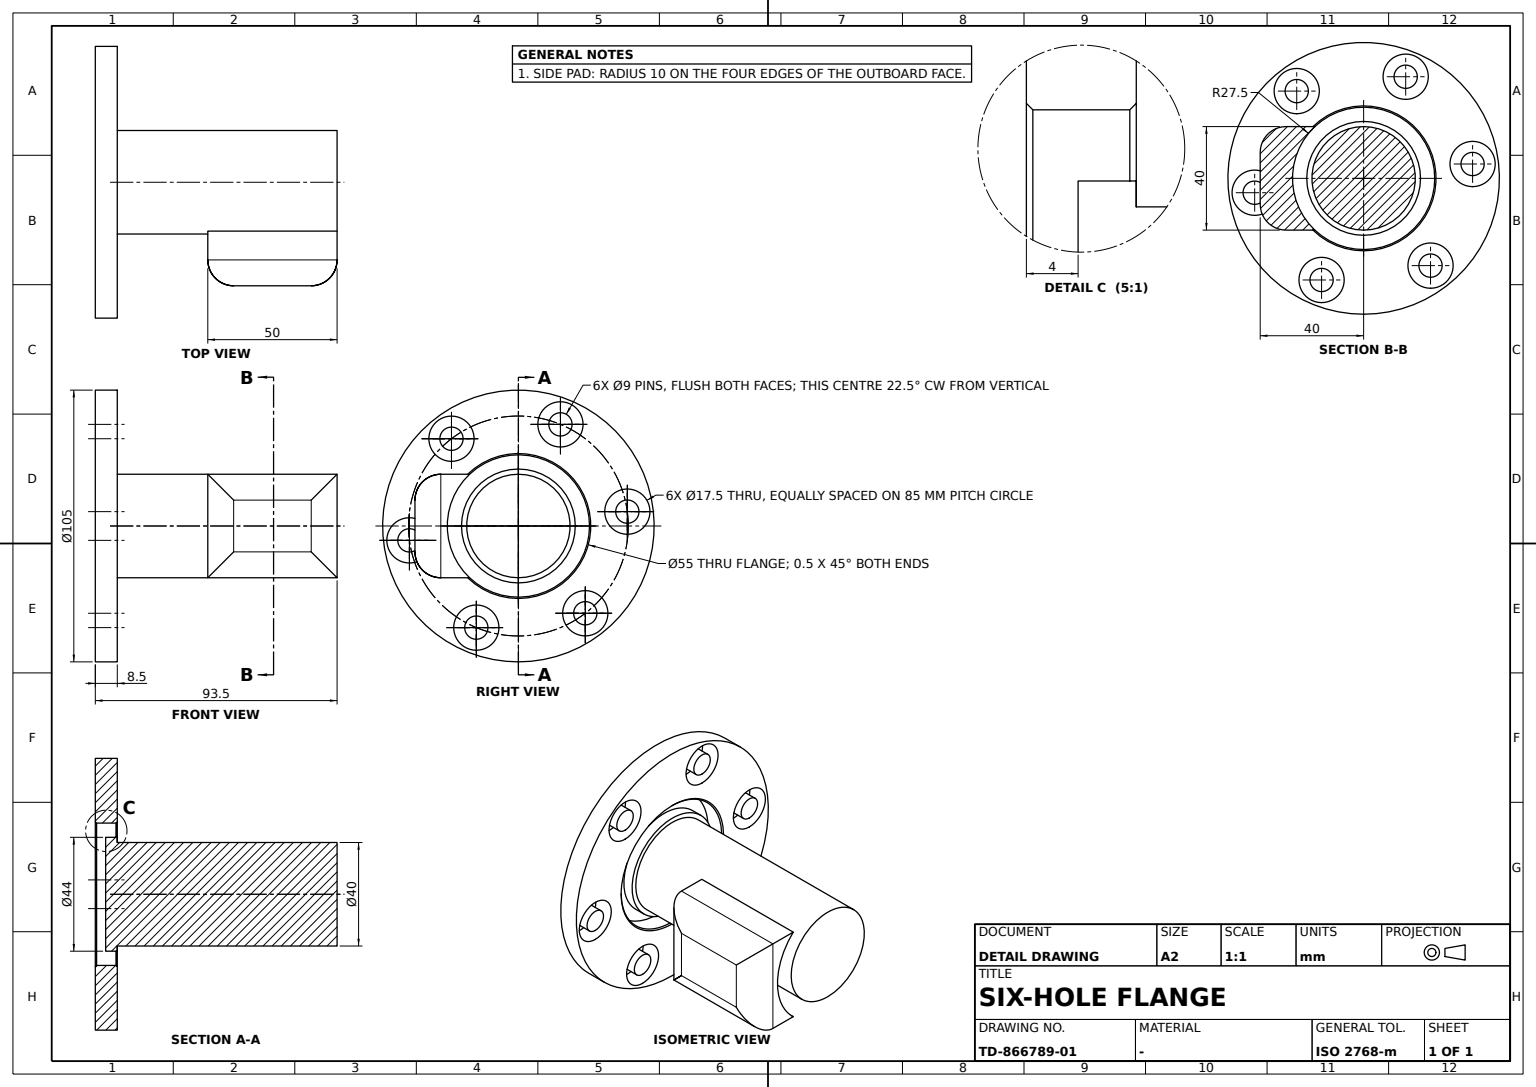
ISO-10303-21;
HEADER;
FILE_DESCRIPTION((''),'2;1');
FILE_NAME('','',(''),(''),'','','');
FILE_SCHEMA(('AUTOMOTIVE_DESIGN'));
ENDSEC;
DATA;
#1=APPLICATION_CONTEXT('');
#2=PRODUCT_CONTEXT('',#1,'mechanical');
#3=PRODUCT('','','',(#2));
#4=PRODUCT_DEFINITION_FORMATION('','',#3);
#5=PRODUCT_DEFINITION_CONTEXT('',#1,'design');
#6=PRODUCT_DEFINITION('','',#4,#5);
#7=PRODUCT_DEFINITION_SHAPE('','',#6);
#8=(LENGTH_UNIT()NAMED_UNIT(*)SI_UNIT(.MILLI.,.METRE.));
#9=(NAMED_UNIT(*)PLANE_ANGLE_UNIT()SI_UNIT($,.RADIAN.));
#10=(NAMED_UNIT(*)SI_UNIT($,.STERADIAN.)SOLID_ANGLE_UNIT());
#11=UNCERTAINTY_MEASURE_WITH_UNIT(LENGTH_MEASURE(0.005),#8,'distance_accuracy_value','');
#12=(GEOMETRIC_REPRESENTATION_CONTEXT(3)GLOBAL_UNCERTAINTY_ASSIGNED_CONTEXT((#11))GLOBAL_UNIT_ASSIGNED_CONTEXT((#8,#9,#10))REPRESENTATION_CONTEXT('',''));
#13=CARTESIAN_POINT('',(-1.047363,42.136407,0.));
#14=VERTEX_POINT('',#13);
#15=CARTESIAN_POINT('',(-5.547363,42.136407,0.));
#16=DIRECTION('',(0.,0.,1.));
#17=DIRECTION('',(1.,0.,0.));
#18=AXIS2_PLACEMENT_3D('',#15,#16,#17);
#19=CIRCLE('',#18,4.5);
#20=EDGE_CURVE('',#14,#14,#19,.T.);
#21=ORIENTED_EDGE('',*,*,#20,.T.);
#22=EDGE_LOOP('',(#21));
#23=FACE_BOUND('',#22,.T.);
#24=CARTESIAN_POINT('',(-1.047363,42.136407,8.5));
#25=VERTEX_POINT('',#24);
#26=CARTESIAN_POINT('',(-5.547363,42.136407,8.5));
#27=AXIS2_PLACEMENT_3D('',#26,#16,#17);
#28=CIRCLE('',#27,4.5);
#29=EDGE_CURVE('',#25,#25,#28,.T.);
#30=ORIENTED_EDGE('',*,*,#29,.F.);
#31=EDGE_LOOP('',(#30));
#32=FACE_BOUND('',#31,.T.);
#33=CARTESIAN_POINT('',(-5.547363,42.136407,4.25));
#34=AXIS2_PLACEMENT_3D('',#33,#16,#17);
#35=CYLINDRICAL_SURFACE('',#34,4.5);
#36=ADVANCED_FACE('',(#23,#32),#35,.T.);
#37=ORIENTED_EDGE('',*,*,#20,.F.);
#38=EDGE_LOOP('',(#37));
#39=FACE_BOUND('',#38,.T.);
#40=CARTESIAN_POINT('',(0.,0.,0.));
#41=AXIS2_PLACEMENT_3D('',#40,#16,#17);
#42=PLANE('',#41);
#43=ADVANCED_FACE('',(#39),#42,.F.);
#44=ORIENTED_EDGE('',*,*,#29,.T.);
#45=EDGE_LOOP('',(#44));
#46=FACE_BOUND('',#45,.T.);
#47=CARTESIAN_POINT('',(0.,0.,8.5));
#48=AXIS2_PLACEMENT_3D('',#47,#16,#17);
#49=PLANE('',#48);
#50=ADVANCED_FACE('',(#46),#49,.T.);
#51=CLOSED_SHELL('',(#36,#43,#50));
#52=MANIFOLD_SOLID_BREP('',#51);
#53=CARTESIAN_POINT('',(52.5,0.,8.5));
#54=VERTEX_POINT('',#53);
#55=CIRCLE('',#48,52.5);
#56=EDGE_CURVE('',#54,#54,#55,.T.);
#57=ORIENTED_EDGE('',*,*,#56,.F.);
#58=EDGE_LOOP('',(#57));
#59=FACE_BOUND('',#58,.T.);
#60=CARTESIAN_POINT('',(52.5,0.,0.));
#61=VERTEX_POINT('',#60);
#62=CIRCLE('',#41,52.5);
#63=EDGE_CURVE('',#61,#61,#62,.T.);
#64=ORIENTED_EDGE('',*,*,#63,.T.);
#65=EDGE_LOOP('',(#64));
#66=FACE_BOUND('',#65,.T.);
#67=CARTESIAN_POINT('',(0.,0.,4.25));
#68=AXIS2_PLACEMENT_3D('',#67,#16,#17);
#69=CYLINDRICAL_SURFACE('',#68,52.5);
#70=ADVANCED_FACE('',(#59,#66),#69,.T.);
#71=CARTESIAN_POINT('',(-30.51488,16.264046,8.5));
#72=VERTEX_POINT('',#71);
#73=CARTESIAN_POINT('',(-39.26488,16.264046,8.5));
#74=AXIS2_PLACEMENT_3D('',#73,#16,#17);
#75=CIRCLE('',#74,8.75);
#76=EDGE_CURVE('',#72,#72,#75,.T.);
#77=ORIENTED_EDGE('',*,*,#76,.T.);
#78=EDGE_LOOP('',(#77));
#79=FACE_BOUND('',#78,.T.);
#80=CARTESIAN_POINT('',(-30.51488,16.264046,0.));
#81=VERTEX_POINT('',#80);
#82=CARTESIAN_POINT('',(-39.26488,16.264046,0.));
#83=AXIS2_PLACEMENT_3D('',#82,#16,#17);
#84=CIRCLE('',#83,8.75);
#85=EDGE_CURVE('',#81,#81,#84,.T.);
#86=ORIENTED_EDGE('',*,*,#85,.F.);
#87=EDGE_LOOP('',(#86));
#88=FACE_BOUND('',#87,.T.);
#89=CARTESIAN_POINT('',(-39.26488,16.264046,4.25));
#90=AXIS2_PLACEMENT_3D('',#89,#16,#17);
#91=CYLINDRICAL_SURFACE('',#90,8.75);
#92=ADVANCED_FACE('',(#79,#88),#91,.F.);
#93=CARTESIAN_POINT('',(0.,-27.5,8.));
#94=VERTEX_POINT('',#93);
#95=CARTESIAN_POINT('',(0.,0.,8.));
#96=DIRECTION('',(0.,-1.,0.));
#97=AXIS2_PLACEMENT_3D('',#95,#16,#96);
#98=CIRCLE('',#97,27.5);
#99=EDGE_CURVE('',#94,#94,#98,.T.);
#100=ORIENTED_EDGE('',*,*,#99,.F.);
#101=EDGE_LOOP('',(#100));
#102=FACE_BOUND('',#101,.T.);
#103=CARTESIAN_POINT('',(28.,0.,8.5));
#104=VERTEX_POINT('',#103);
#105=CIRCLE('',#48,28.);
#106=EDGE_CURVE('',#104,#104,#105,.T.);
#107=ORIENTED_EDGE('',*,*,#106,.T.);
#108=EDGE_LOOP('',(#107));
#109=FACE_BOUND('',#108,.T.);
#110=CARTESIAN_POINT('',(0.,0.,-19.5));
#111=DIRECTION('',(-0.904494219,0.426485883,0.));
#112=AXIS2_PLACEMENT_3D('',#110,#16,#111);
#113=CONICAL_SURFACE('',#112,0.,0.785398163);
#114=ADVANCED_FACE('',(#102,#109),#113,.F.);
#115=ORIENTED_EDGE('',*,*,#56,.T.);
#116=EDGE_LOOP('',(#115));
#117=FACE_BOUND('',#116,.T.);
#118=CARTESIAN_POINT('',(48.01488,-16.264046,8.5));
#119=VERTEX_POINT('',#118);
#120=CARTESIAN_POINT('',(39.26488,-16.264046,8.5));
#121=AXIS2_PLACEMENT_3D('',#120,#16,#17);
#122=CIRCLE('',#121,8.75);
#123=EDGE_CURVE('',#119,#119,#122,.T.);
#124=ORIENTED_EDGE('',*,*,#123,.F.);
#125=EDGE_LOOP('',(#124));
#126=FACE_BOUND('',#125,.T.);
#127=CARTESIAN_POINT('',(3.202637,42.136407,8.5));
#128=VERTEX_POINT('',#127);
#129=CIRCLE('',#27,8.75);
#130=EDGE_CURVE('',#128,#128,#129,.T.);
#131=ORIENTED_EDGE('',*,*,#130,.F.);
#132=EDGE_LOOP('',(#131));
#133=FACE_BOUND('',#132,.T.);
#134=CARTESIAN_POINT('',(14.297363,-42.136407,8.5));
#135=VERTEX_POINT('',#134);
#136=CARTESIAN_POINT('',(5.547363,-42.136407,8.5));
#137=AXIS2_PLACEMENT_3D('',#136,#16,#17);
#138=CIRCLE('',#137,8.75);
#139=EDGE_CURVE('',#135,#135,#138,.T.);
#140=ORIENTED_EDGE('',*,*,#139,.F.);
#141=EDGE_LOOP('',(#140));
#142=FACE_BOUND('',#141,.T.);
#143=ORIENTED_EDGE('',*,*,#76,.F.);
#144=EDGE_LOOP('',(#143));
#145=FACE_BOUND('',#144,.T.);
#146=ORIENTED_EDGE('',*,*,#106,.F.);
#147=EDGE_LOOP('',(#146));
#148=FACE_BOUND('',#147,.T.);
#149=CARTESIAN_POINT('',(42.467517,25.872361,8.5));
#150=VERTEX_POINT('',#149);
#151=CARTESIAN_POINT('',(33.717517,25.872361,8.5));
#152=AXIS2_PLACEMENT_3D('',#151,#16,#17);
#153=CIRCLE('',#152,8.75);
#154=EDGE_CURVE('',#150,#150,#153,.T.);
#155=ORIENTED_EDGE('',*,*,#154,.F.);
#156=EDGE_LOOP('',(#155));
#157=FACE_BOUND('',#156,.T.);
#158=CARTESIAN_POINT('',(-24.967517,-25.872361,8.5));
#159=VERTEX_POINT('',#158);
#160=CARTESIAN_POINT('',(-33.717517,-25.872361,8.5));
#161=AXIS2_PLACEMENT_3D('',#160,#16,#17);
#162=CIRCLE('',#161,8.75);
#163=EDGE_CURVE('',#159,#159,#162,.T.);
#164=ORIENTED_EDGE('',*,*,#163,.F.);
#165=EDGE_LOOP('',(#164));
#166=FACE_BOUND('',#165,.T.);
#167=ADVANCED_FACE('',(#117,#126,#133,#142,#145,#148,#157,#166),#49,.T.);
#168=ORIENTED_EDGE('',*,*,#163,.T.);
#169=EDGE_LOOP('',(#168));
#170=FACE_BOUND('',#169,.T.);
#171=CARTESIAN_POINT('',(-24.967517,-25.872361,0.));
#172=VERTEX_POINT('',#171);
#173=CARTESIAN_POINT('',(-33.717517,-25.872361,0.));
#174=AXIS2_PLACEMENT_3D('',#173,#16,#17);
#175=CIRCLE('',#174,8.75);
#176=EDGE_CURVE('',#172,#172,#175,.T.);
#177=ORIENTED_EDGE('',*,*,#176,.F.);
#178=EDGE_LOOP('',(#177));
#179=FACE_BOUND('',#178,.T.);
#180=CARTESIAN_POINT('',(-33.717517,-25.872361,4.25));
#181=AXIS2_PLACEMENT_3D('',#180,#16,#17);
#182=CYLINDRICAL_SURFACE('',#181,8.75);
#183=ADVANCED_FACE('',(#170,#179),#182,.F.);
#184=ORIENTED_EDGE('',*,*,#130,.T.);
#185=EDGE_LOOP('',(#184));
#186=FACE_BOUND('',#185,.T.);
#187=CARTESIAN_POINT('',(3.202637,42.136407,0.));
#188=VERTEX_POINT('',#187);
#189=CIRCLE('',#18,8.75);
#190=EDGE_CURVE('',#188,#188,#189,.T.);
#191=ORIENTED_EDGE('',*,*,#190,.F.);
#192=EDGE_LOOP('',(#191));
#193=FACE_BOUND('',#192,.T.);
#194=CYLINDRICAL_SURFACE('',#34,8.75);
#195=ADVANCED_FACE('',(#186,#193),#194,.F.);
#196=CARTESIAN_POINT('',(48.01488,-16.264046,0.));
#197=VERTEX_POINT('',#196);
#198=CARTESIAN_POINT('',(39.26488,-16.264046,0.));
#199=AXIS2_PLACEMENT_3D('',#198,#16,#17);
#200=CIRCLE('',#199,8.75);
#201=EDGE_CURVE('',#197,#197,#200,.T.);
#202=ORIENTED_EDGE('',*,*,#201,.F.);
#203=EDGE_LOOP('',(#202));
#204=FACE_BOUND('',#203,.T.);
#205=ORIENTED_EDGE('',*,*,#123,.T.);
#206=EDGE_LOOP('',(#205));
#207=FACE_BOUND('',#206,.T.);
#208=CARTESIAN_POINT('',(39.26488,-16.264046,4.25));
#209=AXIS2_PLACEMENT_3D('',#208,#16,#17);
#210=CYLINDRICAL_SURFACE('',#209,8.75);
#211=ADVANCED_FACE('',(#204,#207),#210,.F.);
#212=ORIENTED_EDGE('',*,*,#190,.T.);
#213=EDGE_LOOP('',(#212));
#214=FACE_BOUND('',#213,.T.);
#215=ORIENTED_EDGE('',*,*,#85,.T.);
#216=EDGE_LOOP('',(#215));
#217=FACE_BOUND('',#216,.T.);
#218=ORIENTED_EDGE('',*,*,#63,.F.);
#219=EDGE_LOOP('',(#218));
#220=FACE_BOUND('',#219,.T.);
#221=ORIENTED_EDGE('',*,*,#201,.T.);
#222=EDGE_LOOP('',(#221));
#223=FACE_BOUND('',#222,.T.);
#224=CARTESIAN_POINT('',(42.467517,25.872361,0.));
#225=VERTEX_POINT('',#224);
#226=CARTESIAN_POINT('',(33.717517,25.872361,0.));
#227=AXIS2_PLACEMENT_3D('',#226,#16,#17);
#228=CIRCLE('',#227,8.75);
#229=EDGE_CURVE('',#225,#225,#228,.T.);
#230=ORIENTED_EDGE('',*,*,#229,.T.);
#231=EDGE_LOOP('',(#230));
#232=FACE_BOUND('',#231,.T.);
#233=CARTESIAN_POINT('',(28.,0.,0.));
#234=VERTEX_POINT('',#233);
#235=CIRCLE('',#41,28.);
#236=EDGE_CURVE('',#234,#234,#235,.T.);
#237=ORIENTED_EDGE('',*,*,#236,.T.);
#238=EDGE_LOOP('',(#237));
#239=FACE_BOUND('',#238,.T.);
#240=CARTESIAN_POINT('',(14.297363,-42.136407,0.));
#241=VERTEX_POINT('',#240);
#242=CARTESIAN_POINT('',(5.547363,-42.136407,0.));
#243=AXIS2_PLACEMENT_3D('',#242,#16,#17);
#244=CIRCLE('',#243,8.75);
#245=EDGE_CURVE('',#241,#241,#244,.T.);
#246=ORIENTED_EDGE('',*,*,#245,.T.);
#247=EDGE_LOOP('',(#246));
#248=FACE_BOUND('',#247,.T.);
#249=ORIENTED_EDGE('',*,*,#176,.T.);
#250=EDGE_LOOP('',(#249));
#251=FACE_BOUND('',#250,.T.);
#252=ADVANCED_FACE('',(#214,#217,#220,#223,#232,#239,#248,#251),#42,.F.);
#253=ORIENTED_EDGE('',*,*,#236,.F.);
#254=EDGE_LOOP('',(#253));
#255=FACE_BOUND('',#254,.T.);
#256=CARTESIAN_POINT('',(0.,27.5,0.5));
#257=VERTEX_POINT('',#256);
#258=CARTESIAN_POINT('',(0.,0.,0.5));
#259=DIRECTION('',(0.,0.,-1.));
#260=DIRECTION('',(0.,1.,0.));
#261=AXIS2_PLACEMENT_3D('',#258,#259,#260);
#262=CIRCLE('',#261,27.5);
#263=EDGE_CURVE('',#257,#257,#262,.F.);
#264=ORIENTED_EDGE('',*,*,#263,.T.);
#265=EDGE_LOOP('',(#264));
#266=FACE_BOUND('',#265,.T.);
#267=CARTESIAN_POINT('',(0.,0.,28.));
#268=DIRECTION('',(0.904494219,-0.426485883,0.));
#269=AXIS2_PLACEMENT_3D('',#267,#259,#268);
#270=CONICAL_SURFACE('',#269,0.,0.785398163);
#271=ADVANCED_FACE('',(#255,#266),#270,.F.);
#272=ORIENTED_EDGE('',*,*,#229,.F.);
#273=EDGE_LOOP('',(#272));
#274=FACE_BOUND('',#273,.T.);
#275=ORIENTED_EDGE('',*,*,#154,.T.);
#276=EDGE_LOOP('',(#275));
#277=FACE_BOUND('',#276,.T.);
#278=CARTESIAN_POINT('',(33.717517,25.872361,4.25));
#279=AXIS2_PLACEMENT_3D('',#278,#16,#17);
#280=CYLINDRICAL_SURFACE('',#279,8.75);
#281=ADVANCED_FACE('',(#274,#277),#280,.F.);
#282=ORIENTED_EDGE('',*,*,#263,.F.);
#283=EDGE_LOOP('',(#282));
#284=FACE_BOUND('',#283,.T.);
#285=ORIENTED_EDGE('',*,*,#99,.T.);
#286=EDGE_LOOP('',(#285));
#287=FACE_BOUND('',#286,.T.);
#288=CYLINDRICAL_SURFACE('',#68,27.5);
#289=ADVANCED_FACE('',(#284,#287),#288,.F.);
#290=ORIENTED_EDGE('',*,*,#139,.T.);
#291=EDGE_LOOP('',(#290));
#292=FACE_BOUND('',#291,.T.);
#293=ORIENTED_EDGE('',*,*,#245,.F.);
#294=EDGE_LOOP('',(#293));
#295=FACE_BOUND('',#294,.T.);
#296=CARTESIAN_POINT('',(5.547363,-42.136407,4.25));
#297=AXIS2_PLACEMENT_3D('',#296,#16,#17);
#298=CYLINDRICAL_SURFACE('',#297,8.75);
#299=ADVANCED_FACE('',(#292,#295),#298,.F.);
#300=CLOSED_SHELL('',(#70,#92,#114,#167,#183,#195,#211,#252,#271,#281,#289,#299));
#301=MANIFOLD_SOLID_BREP('',#300);
#302=CARTESIAN_POINT('',(22.,0.,4.));
#303=VERTEX_POINT('',#302);
#304=CARTESIAN_POINT('',(0.,0.,4.));
#305=AXIS2_PLACEMENT_3D('',#304,#16,#17);
#306=CIRCLE('',#305,22.);
#307=EDGE_CURVE('',#303,#303,#306,.T.);
#308=ORIENTED_EDGE('',*,*,#307,.T.);
#309=EDGE_LOOP('',(#308));
#310=FACE_BOUND('',#309,.T.);
#311=CARTESIAN_POINT('',(22.,0.,8.5));
#312=VERTEX_POINT('',#311);
#313=CIRCLE('',#48,22.);
#314=EDGE_CURVE('',#312,#312,#313,.T.);
#315=ORIENTED_EDGE('',*,*,#314,.F.);
#316=EDGE_LOOP('',(#315));
#317=FACE_BOUND('',#316,.T.);
#318=CYLINDRICAL_SURFACE('',#68,22.);
#319=ADVANCED_FACE('',(#310,#317),#318,.T.);
#320=CARTESIAN_POINT('',(20.,0.,93.5));
#321=VERTEX_POINT('',#320);
#322=CARTESIAN_POINT('',(0.,0.,93.5));
#323=AXIS2_PLACEMENT_3D('',#322,#16,#17);
#324=CIRCLE('',#323,20.);
#325=EDGE_CURVE('',#321,#321,#324,.T.);
#326=ORIENTED_EDGE('',*,*,#325,.T.);
#327=EDGE_LOOP('',(#326));
#328=FACE_BOUND('',#327,.T.);
#329=PLANE('',#323);
#330=ADVANCED_FACE('',(#328),#329,.T.);
#331=ORIENTED_EDGE('',*,*,#314,.T.);
#332=EDGE_LOOP('',(#331));
#333=FACE_BOUND('',#332,.T.);
#334=CARTESIAN_POINT('',(20.,0.,8.5));
#335=VERTEX_POINT('',#334);
#336=CIRCLE('',#48,20.);
#337=EDGE_CURVE('',#335,#335,#336,.T.);
#338=ORIENTED_EDGE('',*,*,#337,.F.);
#339=EDGE_LOOP('',(#338));
#340=FACE_BOUND('',#339,.T.);
#341=ADVANCED_FACE('',(#333,#340),#49,.T.);
#342=ORIENTED_EDGE('',*,*,#337,.T.);
#343=EDGE_LOOP('',(#342));
#344=FACE_BOUND('',#343,.T.);
#345=ORIENTED_EDGE('',*,*,#325,.F.);
#346=EDGE_LOOP('',(#345));
#347=FACE_BOUND('',#346,.T.);
#348=CARTESIAN_POINT('',(0.,0.,51.));
#349=AXIS2_PLACEMENT_3D('',#348,#16,#17);
#350=CYLINDRICAL_SURFACE('',#349,20.);
#351=ADVANCED_FACE('',(#344,#347),#350,.T.);
#352=ORIENTED_EDGE('',*,*,#307,.F.);
#353=EDGE_LOOP('',(#352));
#354=FACE_BOUND('',#353,.T.);
#355=CARTESIAN_POINT('',(-1.616457,0.,4.));
#356=AXIS2_PLACEMENT_3D('',#355,#16,#17);
#357=PLANE('',#356);
#358=ADVANCED_FACE('',(#354),#357,.F.);
#359=CLOSED_SHELL('',(#319,#330,#341,#351,#358));
#360=MANIFOLD_SOLID_BREP('',#359);
#361=CARTESIAN_POINT('',(38.217517,25.872361,0.));
#362=VERTEX_POINT('',#361);
#363=CIRCLE('',#227,4.5);
#364=EDGE_CURVE('',#362,#362,#363,.T.);
#365=ORIENTED_EDGE('',*,*,#364,.F.);
#366=EDGE_LOOP('',(#365));
#367=FACE_BOUND('',#366,.T.);
#368=ADVANCED_FACE('',(#367),#42,.F.);
#369=CARTESIAN_POINT('',(38.217517,25.872361,8.5));
#370=VERTEX_POINT('',#369);
#371=CIRCLE('',#152,4.5);
#372=EDGE_CURVE('',#370,#370,#371,.T.);
#373=ORIENTED_EDGE('',*,*,#372,.T.);
#374=EDGE_LOOP('',(#373));
#375=FACE_BOUND('',#374,.T.);
#376=ADVANCED_FACE('',(#375),#49,.T.);
#377=ORIENTED_EDGE('',*,*,#364,.T.);
#378=EDGE_LOOP('',(#377));
#379=FACE_BOUND('',#378,.T.);
#380=ORIENTED_EDGE('',*,*,#372,.F.);
#381=EDGE_LOOP('',(#380));
#382=FACE_BOUND('',#381,.T.);
#383=CYLINDRICAL_SURFACE('',#279,4.5);
#384=ADVANCED_FACE('',(#379,#382),#383,.T.);
#385=CLOSED_SHELL('',(#368,#376,#384));
#386=MANIFOLD_SOLID_BREP('',#385);
#387=CARTESIAN_POINT('',(43.76488,-16.264046,8.5));
#388=VERTEX_POINT('',#387);
#389=CIRCLE('',#121,4.5);
#390=EDGE_CURVE('',#388,#388,#389,.T.);
#391=ORIENTED_EDGE('',*,*,#390,.F.);
#392=EDGE_LOOP('',(#391));
#393=FACE_BOUND('',#392,.T.);
#394=CARTESIAN_POINT('',(43.76488,-16.264046,0.));
#395=VERTEX_POINT('',#394);
#396=CIRCLE('',#199,4.5);
#397=EDGE_CURVE('',#395,#395,#396,.T.);
#398=ORIENTED_EDGE('',*,*,#397,.T.);
#399=EDGE_LOOP('',(#398));
#400=FACE_BOUND('',#399,.T.);
#401=CYLINDRICAL_SURFACE('',#209,4.5);
#402=ADVANCED_FACE('',(#393,#400),#401,.T.);
#403=ORIENTED_EDGE('',*,*,#390,.T.);
#404=EDGE_LOOP('',(#403));
#405=FACE_BOUND('',#404,.T.);
#406=ADVANCED_FACE('',(#405),#49,.T.);
#407=ORIENTED_EDGE('',*,*,#397,.F.);
#408=EDGE_LOOP('',(#407));
#409=FACE_BOUND('',#408,.T.);
#410=ADVANCED_FACE('',(#409),#42,.F.);
#411=CLOSED_SHELL('',(#402,#406,#410));
#412=MANIFOLD_SOLID_BREP('',#411);
#413=CARTESIAN_POINT('',(10.047363,-42.136407,8.5));
#414=VERTEX_POINT('',#413);
#415=CIRCLE('',#137,4.5);
#416=EDGE_CURVE('',#414,#414,#415,.T.);
#417=ORIENTED_EDGE('',*,*,#416,.T.);
#418=EDGE_LOOP('',(#417));
#419=FACE_BOUND('',#418,.T.);
#420=ADVANCED_FACE('',(#419),#49,.T.);
#421=ORIENTED_EDGE('',*,*,#416,.F.);
#422=EDGE_LOOP('',(#421));
#423=FACE_BOUND('',#422,.T.);
#424=CARTESIAN_POINT('',(10.047363,-42.136407,0.));
#425=VERTEX_POINT('',#424);
#426=CIRCLE('',#243,4.5);
#427=EDGE_CURVE('',#425,#425,#426,.T.);
#428=ORIENTED_EDGE('',*,*,#427,.T.);
#429=EDGE_LOOP('',(#428));
#430=FACE_BOUND('',#429,.T.);
#431=CYLINDRICAL_SURFACE('',#297,4.5);
#432=ADVANCED_FACE('',(#423,#430),#431,.T.);
#433=ORIENTED_EDGE('',*,*,#427,.F.);
#434=EDGE_LOOP('',(#433));
#435=FACE_BOUND('',#434,.T.);
#436=ADVANCED_FACE('',(#435),#42,.F.);
#437=CLOSED_SHELL('',(#420,#432,#436));
#438=MANIFOLD_SOLID_BREP('',#437);
#439=CARTESIAN_POINT('',(-29.217517,-25.872361,0.));
#440=VERTEX_POINT('',#439);
#441=CIRCLE('',#174,4.5);
#442=EDGE_CURVE('',#440,#440,#441,.T.);
#443=ORIENTED_EDGE('',*,*,#442,.T.);
#444=EDGE_LOOP('',(#443));
#445=FACE_BOUND('',#444,.T.);
#446=CARTESIAN_POINT('',(-29.217517,-25.872361,8.5));
#447=VERTEX_POINT('',#446);
#448=CIRCLE('',#161,4.5);
#449=EDGE_CURVE('',#447,#447,#448,.T.);
#450=ORIENTED_EDGE('',*,*,#449,.F.);
#451=EDGE_LOOP('',(#450));
#452=FACE_BOUND('',#451,.T.);
#453=CYLINDRICAL_SURFACE('',#181,4.5);
#454=ADVANCED_FACE('',(#445,#452),#453,.T.);
#455=ORIENTED_EDGE('',*,*,#449,.T.);
#456=EDGE_LOOP('',(#455));
#457=FACE_BOUND('',#456,.T.);
#458=ADVANCED_FACE('',(#457),#49,.T.);
#459=ORIENTED_EDGE('',*,*,#442,.F.);
#460=EDGE_LOOP('',(#459));
#461=FACE_BOUND('',#460,.T.);
#462=ADVANCED_FACE('',(#461),#42,.F.);
#463=CLOSED_SHELL('',(#454,#458,#462));
#464=MANIFOLD_SOLID_BREP('',#463);
#465=CARTESIAN_POINT('',(-34.76488,16.264046,8.5));
#466=VERTEX_POINT('',#465);
#467=CIRCLE('',#74,4.5);
#468=EDGE_CURVE('',#466,#466,#467,.T.);
#469=ORIENTED_EDGE('',*,*,#468,.T.);
#470=EDGE_LOOP('',(#469));
#471=FACE_BOUND('',#470,.T.);
#472=ADVANCED_FACE('',(#471),#49,.T.);
#473=CARTESIAN_POINT('',(-34.76488,16.264046,0.));
#474=VERTEX_POINT('',#473);
#475=CIRCLE('',#83,4.5);
#476=EDGE_CURVE('',#474,#474,#475,.T.);
#477=ORIENTED_EDGE('',*,*,#476,.T.);
#478=EDGE_LOOP('',(#477));
#479=FACE_BOUND('',#478,.T.);
#480=ORIENTED_EDGE('',*,*,#468,.F.);
#481=EDGE_LOOP('',(#480));
#482=FACE_BOUND('',#481,.T.);
#483=CYLINDRICAL_SURFACE('',#90,4.5);
#484=ADVANCED_FACE('',(#479,#482),#483,.T.);
#485=ORIENTED_EDGE('',*,*,#476,.F.);
#486=EDGE_LOOP('',(#485));
#487=FACE_BOUND('',#486,.T.);
#488=ADVANCED_FACE('',(#487),#42,.F.);
#489=CLOSED_SHELL('',(#472,#484,#488));
#490=MANIFOLD_SOLID_BREP('',#489);
#491=CARTESIAN_POINT('',(-10.,-40.,53.5));
#492=VERTEX_POINT('',#491);
#493=CARTESIAN_POINT('',(-20.,-30.,43.5));
#494=VERTEX_POINT('',#493);
#495=CARTESIAN_POINT('',(-10.,-30.,53.5));
#496=DIRECTION('',(0.707106781,0.,-0.707106781));
#497=DIRECTION('',(0.707106781,0.,0.707106781));
#498=AXIS2_PLACEMENT_3D('',#495,#496,#497);
#499=ELLIPSE('',#498,14.142136,10.);
#500=EDGE_CURVE('',#492,#494,#499,.T.);
#501=ORIENTED_EDGE('',*,*,#500,.T.);
#502=CARTESIAN_POINT('',(20.,-30.,43.5));
#503=VERTEX_POINT('',#502);
#504=CARTESIAN_POINT('',(0.,-30.,43.5));
#505=VECTOR('',#17,1000.);
#506=LINE('',#504,#505);
#507=EDGE_CURVE('',#494,#503,#506,.T.);
#508=ORIENTED_EDGE('',*,*,#507,.T.);
#509=CARTESIAN_POINT('',(10.,-40.,53.5));
#510=VERTEX_POINT('',#509);
#511=CARTESIAN_POINT('',(10.,-30.,53.5));
#512=DIRECTION('',(-0.707106781,0.,-0.707106781));
#513=AXIS2_PLACEMENT_3D('',#511,#512,#496);
#514=ELLIPSE('',#513,14.142136,10.);
#515=EDGE_CURVE('',#510,#503,#514,.F.);
#516=ORIENTED_EDGE('',*,*,#515,.F.);
#517=CARTESIAN_POINT('',(0.,-40.,53.5));
#518=LINE('',#517,#505);
#519=EDGE_CURVE('',#492,#510,#518,.T.);
#520=ORIENTED_EDGE('',*,*,#519,.F.);
#521=EDGE_LOOP('',(#501,#508,#516,#520));
#522=FACE_BOUND('',#521,.T.);
#523=CARTESIAN_POINT('',(0.,-30.,53.5));
#524=AXIS2_PLACEMENT_3D('',#523,#17,#96);
#525=CYLINDRICAL_SURFACE('',#524,10.);
#526=ADVANCED_FACE('',(#522),#525,.T.);
#527=CARTESIAN_POINT('',(20.,-18.874586,43.5));
#528=VERTEX_POINT('',#527);
#529=VECTOR('',#96,1000.);
#530=LINE('',#527,#529);
#531=EDGE_CURVE('',#528,#503,#530,.T.);
#532=ORIENTED_EDGE('',*,*,#531,.T.);
#533=ORIENTED_EDGE('',*,*,#507,.F.);
#534=CARTESIAN_POINT('',(-20.,-18.874586,43.5));
#535=VERTEX_POINT('',#534);
#536=CARTESIAN_POINT('',(-20.,-40.,43.5));
#537=VECTOR('',#260,1000.);
#538=LINE('',#536,#537);
#539=EDGE_CURVE('',#494,#535,#538,.T.);
#540=ORIENTED_EDGE('',*,*,#539,.T.);
#541=CARTESIAN_POINT('',(0.,0.,43.5));
#542=AXIS2_PLACEMENT_3D('',#541,#16,#17);
#543=CIRCLE('',#542,27.5);
#544=EDGE_CURVE('',#535,#528,#543,.T.);
#545=ORIENTED_EDGE('',*,*,#544,.T.);
#546=EDGE_LOOP('',(#532,#533,#540,#545));
#547=FACE_BOUND('',#546,.T.);
#548=PLANE('',#542);
#549=ADVANCED_FACE('',(#547),#548,.F.);
#550=CARTESIAN_POINT('',(-20.,-30.,93.5));
#551=VERTEX_POINT('',#550);
#552=CARTESIAN_POINT('',(-20.,-18.874586,93.5));
#553=VERTEX_POINT('',#552);
#554=CARTESIAN_POINT('',(-20.,-40.,93.5));
#555=LINE('',#554,#537);
#556=EDGE_CURVE('',#551,#553,#555,.T.);
#557=ORIENTED_EDGE('',*,*,#556,.F.);
#558=CARTESIAN_POINT('',(20.,-30.,93.5));
#559=VERTEX_POINT('',#558);
#560=CARTESIAN_POINT('',(0.,-30.,93.5));
#561=LINE('',#560,#505);
#562=EDGE_CURVE('',#551,#559,#561,.T.);
#563=ORIENTED_EDGE('',*,*,#562,.T.);
#564=CARTESIAN_POINT('',(20.,-18.874586,93.5));
#565=VERTEX_POINT('',#564);
#566=LINE('',#564,#529);
#567=EDGE_CURVE('',#565,#559,#566,.T.);
#568=ORIENTED_EDGE('',*,*,#567,.F.);
#569=CIRCLE('',#323,27.5);
#570=EDGE_CURVE('',#553,#565,#569,.T.);
#571=ORIENTED_EDGE('',*,*,#570,.F.);
#572=EDGE_LOOP('',(#557,#563,#568,#571));
#573=FACE_BOUND('',#572,.T.);
#574=ADVANCED_FACE('',(#573),#329,.T.);
#575=ORIENTED_EDGE('',*,*,#500,.F.);
#576=CARTESIAN_POINT('',(-10.,-40.,83.5));
#577=VERTEX_POINT('',#576);
#578=CARTESIAN_POINT('',(-10.,-40.,68.5));
#579=VECTOR('',#259,1000.);
#580=LINE('',#578,#579);
#581=EDGE_CURVE('',#577,#492,#580,.T.);
#582=ORIENTED_EDGE('',*,*,#581,.F.);
#583=CARTESIAN_POINT('',(-10.,-30.,83.5));
#584=AXIS2_PLACEMENT_3D('',#583,#512,#496);
#585=ELLIPSE('',#584,14.142136,10.);
#586=EDGE_CURVE('',#577,#551,#585,.T.);
#587=ORIENTED_EDGE('',*,*,#586,.T.);
#588=CARTESIAN_POINT('',(-20.,-30.,68.5));
#589=LINE('',#588,#579);
#590=EDGE_CURVE('',#551,#494,#589,.T.);
#591=ORIENTED_EDGE('',*,*,#590,.T.);
#592=EDGE_LOOP('',(#575,#582,#587,#591));
#593=FACE_BOUND('',#592,.T.);
#594=CARTESIAN_POINT('',(-10.,-30.,68.5));
#595=AXIS2_PLACEMENT_3D('',#594,#259,#96);
#596=CYLINDRICAL_SURFACE('',#595,10.);
#597=ADVANCED_FACE('',(#593),#596,.T.);
#598=ORIENTED_EDGE('',*,*,#539,.F.);
#599=ORIENTED_EDGE('',*,*,#590,.F.);
#600=ORIENTED_EDGE('',*,*,#556,.T.);
#601=VECTOR('',#16,1000.);
#602=LINE('',#552,#601);
#603=EDGE_CURVE('',#553,#535,#602,.F.);
#604=ORIENTED_EDGE('',*,*,#603,.T.);
#605=EDGE_LOOP('',(#598,#599,#600,#604));
#606=FACE_BOUND('',#605,.T.);
#607=DIRECTION('',(-1.,0.,0.));
#608=AXIS2_PLACEMENT_3D('',#554,#607,#260);
#609=PLANE('',#608);
#610=ADVANCED_FACE('',(#606),#609,.T.);
#611=CARTESIAN_POINT('',(10.,-40.,83.5));
#612=VERTEX_POINT('',#611);
#613=CARTESIAN_POINT('',(10.,-30.,83.5));
#614=AXIS2_PLACEMENT_3D('',#613,#496,#497);
#615=ELLIPSE('',#614,14.142136,10.);
#616=EDGE_CURVE('',#612,#559,#615,.F.);
#617=ORIENTED_EDGE('',*,*,#616,.T.);
#618=ORIENTED_EDGE('',*,*,#562,.F.);
#619=ORIENTED_EDGE('',*,*,#586,.F.);
#620=CARTESIAN_POINT('',(0.,-40.,83.5));
#621=LINE('',#620,#505);
#622=EDGE_CURVE('',#577,#612,#621,.T.);
#623=ORIENTED_EDGE('',*,*,#622,.T.);
#624=EDGE_LOOP('',(#617,#618,#619,#623));
#625=FACE_BOUND('',#624,.T.);
#626=CARTESIAN_POINT('',(0.,-30.,83.5));
#627=AXIS2_PLACEMENT_3D('',#626,#17,#96);
#628=CYLINDRICAL_SURFACE('',#627,10.);
#629=ADVANCED_FACE('',(#625),#628,.T.);
#630=LINE('',#564,#601);
#631=EDGE_CURVE('',#565,#528,#630,.F.);
#632=ORIENTED_EDGE('',*,*,#631,.T.);
#633=ORIENTED_EDGE('',*,*,#544,.F.);
#634=ORIENTED_EDGE('',*,*,#603,.F.);
#635=ORIENTED_EDGE('',*,*,#570,.T.);
#636=EDGE_LOOP('',(#632,#633,#634,#635));
#637=FACE_BOUND('',#636,.T.);
#638=ADVANCED_FACE('',(#637),#288,.F.);
#639=ORIENTED_EDGE('',*,*,#616,.F.);
#640=CARTESIAN_POINT('',(10.,-40.,68.5));
#641=LINE('',#640,#579);
#642=EDGE_CURVE('',#612,#510,#641,.T.);
#643=ORIENTED_EDGE('',*,*,#642,.T.);
#644=ORIENTED_EDGE('',*,*,#515,.T.);
#645=CARTESIAN_POINT('',(20.,-30.,68.5));
#646=LINE('',#645,#579);
#647=EDGE_CURVE('',#559,#503,#646,.T.);
#648=ORIENTED_EDGE('',*,*,#647,.F.);
#649=EDGE_LOOP('',(#639,#643,#644,#648));
#650=FACE_BOUND('',#649,.T.);
#651=CARTESIAN_POINT('',(10.,-30.,68.5));
#652=AXIS2_PLACEMENT_3D('',#651,#259,#96);
#653=CYLINDRICAL_SURFACE('',#652,10.);
#654=ADVANCED_FACE('',(#650),#653,.T.);
#655=ORIENTED_EDGE('',*,*,#519,.T.);
#656=ORIENTED_EDGE('',*,*,#642,.F.);
#657=ORIENTED_EDGE('',*,*,#622,.F.);
#658=ORIENTED_EDGE('',*,*,#581,.T.);
#659=EDGE_LOOP('',(#655,#656,#657,#658));
#660=FACE_BOUND('',#659,.T.);
#661=CARTESIAN_POINT('',(20.,-40.,93.5));
#662=AXIS2_PLACEMENT_3D('',#661,#96,#607);
#663=PLANE('',#662);
#664=ADVANCED_FACE('',(#660),#663,.T.);
#665=ORIENTED_EDGE('',*,*,#647,.T.);
#666=ORIENTED_EDGE('',*,*,#531,.F.);
#667=ORIENTED_EDGE('',*,*,#631,.F.);
#668=ORIENTED_EDGE('',*,*,#567,.T.);
#669=EDGE_LOOP('',(#665,#666,#667,#668));
#670=FACE_BOUND('',#669,.T.);
#671=AXIS2_PLACEMENT_3D('',#564,#17,#96);
#672=PLANE('',#671);
#673=ADVANCED_FACE('',(#670),#672,.T.);
#674=CLOSED_SHELL('',(#526,#549,#574,#597,#610,#629,#638,#654,#664,#673));
#675=MANIFOLD_SOLID_BREP('',#674);
#676=ADVANCED_BREP_SHAPE_REPRESENTATION('',(#52,#301,#360,#386,#412,#438,#464,#490,#675),#12);
#677=SHAPE_DEFINITION_REPRESENTATION(#7,#676);
ENDSEC;
END-ISO-10303-21;
